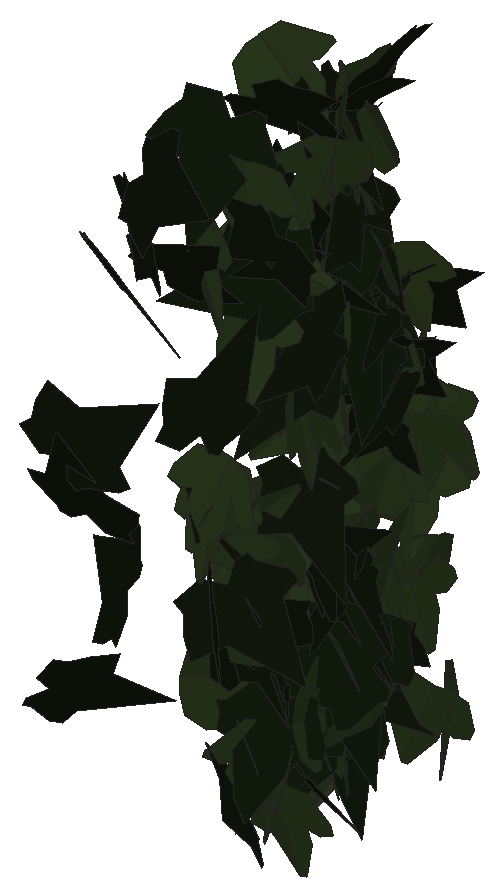
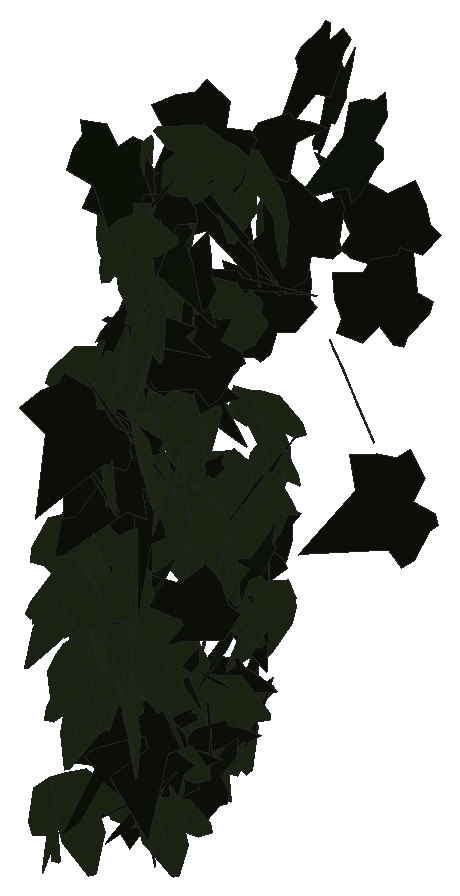
# SketchUp Ruby script. Lengths in inches.
U = 1.inch
M = Sketchup.active_model
def pt(a) = Geom::Point3d.new(a.map { |v| v * U })
def face(e, loops, mat)
  f = e.add_face(loops[0].map { |a| pt(a) })
  loops[1..].each { |l| e.add_face(l.map { |a| pt(a) }).erase! }
  f.material = f.back_material = mat if mat
  f
end
# faces: each face lists its corners as indices into pts; further lists are holes
def faces(e, pts, list, mat = nil) = list.each { |f| face(e, (f[0].is_a?(Array) ? f : [f]).map { |l| l.map { |i| pts[i] } }, mat) }
# xy, xz, yz: faces in a plane at the given z, y or x. An outline is a flat list of corners, or four numbers for a rectangle; further outlines are holes
def ring(l) = l.size == 4 ? [[l[0], l[1]], [l[2], l[1]], [l[2], l[3]], [l[0], l[3]]] : l.each_slice(2).to_a
def flat(e, list, mat, &to3) = list.each { |f| face(e, (f[0].is_a?(Array) ? f : [f]).map { |l| ring(l).map { |u, v| to3.(u, v) } }, mat) }
def xy(e, z, list, mat = nil) = flat(e, list, mat) { |x, y| [x, y, z] }
def xz(e, y, list, mat = nil) = flat(e, list, mat) { |x, z| [x, y, z] }
def yz(e, x, list, mat = nil) = flat(e, list, mat) { |y, z| [x, y, z] }
def lines(e, pts, list) = list.each { |a, b| e.add_line(pt(pts[a]), pt(pts[b])) }
# prism: a flat outline (further loops are holes) pulled along v
def prism(e, loops, v, mat = nil)
  f = face(e, loops, mat); d = Geom::Vector3d.new(v.map { |x| x * U })
  f.pushpull(f.normal.samedirection?(d) ? d.length : -d.length)
end
def box(e, o, s, mat = nil) = prism(e, [[o, [o[0] + s[0], o[1], o[2]], [o[0] + s[0], o[1] + s[1], o[2]], [o[0], o[1] + s[1], o[2]]]], [0, 0, s[2]], mat)
def at(x, y, z, deg = 0) = Geom::Transformation.translation(pt([x, y, z])) * Geom::Transformation.rotation(ORIGIN, Z_AXIS, deg.degrees)
def axes(o, x, y, z) = Geom::Transformation.new([*x, 0, *y, 0, *z, 0, *pt(o).to_a, 1])
def part(name) = M.definitions.add(name)
# library, detail: a bought-in or finely detailed component or shape, given as its bounding box
def library(name, o, s) = part(name).tap { |d| box(d.entities, o, s) }
def detail(e, o, s) = box(e.add_group.entities, o, s)
def put(e, d, t, mat = nil) = e.add_instance(d, t).tap { |i| i.material = mat if mat }
def group(e, t, mat = nil) = e.add_group.tap { |g| g.transformation = t; g.material = mat if mat }.entities
root = M.entities
M.materials.add("efeu1").color = [18, 25, 13]
M.materials.add("efeu2").color = [43, 57, 29]
c1 = part("ivyleaf_9")
p = [[1.54,2.16,1.25],[1.36,2.04,1.19],[-0.21,0.99,0.68],[-0.71,1.11,0.82],[-0.85,0.86,0.67],[-0.8,0.17,0.21],
  [-0.9,-0.01,0.1],[-0.67,-0.16,-0.02],[-0.08,-0.08,-0.05],[-0.03,-0.6,-0.4],[0.65,-0.88,-0.66],[0.83,-0.6,-0.49],
  [1.29,-0.42,-0.43],[1.8125,-0.07,-0.26],[1.21,0.44,0.15]]
faces(c1.entities,p,[[0,1,2,3,4,5,6,7,8,9,10,11,12,13,14]],"efeu1")
c2 = part("ivyleaf_10")
p = [[0,0.5,-0.03],[-0.0625,2.02,-0.43],[-0.19,2.01,-0.46],[-0.54,1.05,-0.29],[-0.52,0.625,-0.18],[-0.83,0.76,-0.28],
  [-1.16,0.64,-0.33],[-1.15,0.33,-0.24],[-0.77,-0.39,0.02],[-0.3,-0.51,0.16],[0.04,-0.48,0.23],[-0.02,2.01,-0.4375],
  [-0.06,2.01,-0.43],[0.04,-0.49,0.23],[0.67,-0.49,0.14],[1.38,0.36,-0.2],[1.375,0.51,-0.24],[0.81,0.65,-0.19],
  [0.62,0.59,-0.15],[0.6,1.09,-0.28],[0.5,1.23,-0.31]]
faces(c2.entities,p,[[0,1,2,3,4,5,6,7,8,9,10],[11,12,0,13,14,15,16,17,18,19,20]],"efeu2")
put(root,c1,axes([54.05,220.4,216.4],[0.34278,0.22043,0.28967],[0.24301,0.15765,-0.40754],[-0.27101,0.42018,0.00094]))
put(root,c2,axes([54.22,224.41,218.67],[-0.03576,-0.11891,-0.48434],[0.01811,-0.48557,0.11788],[-0.49839,-0.00912,0.03904]))
put(root,c2,axes([54.375,225.42,215.87],[0.18568,-0.42925,-0.17682],[-0.07392,0.16068,-0.46767],[0.45832,0.19982,-0.00379]))
put(root,c2,axes([54.09,224.46,218.04],[-0.36251,-0.05995,-0.33911],[0.33393,0.05912,-0.36742],[0.08415,-0.49286,-0.00282]))
put(root,c2,axes([54.24,224.94,214.08],[0.46856,0.17151,-0.03227],[-0.02948,-0.01334,-0.49895],[-0.17201,0.46948,-0.00239]))
put(root,c2,axes([54.38,223.75,215.08],[-0.39712,-0.30366,0.00943],[-0.00588,-0.00784,-0.4999],[0.30375,-0.39715,0.00266]))
put(root,c2,axes([54.36,225.33,217.76],[0.03123,-0.49331,-0.0753],[-0.0092,0.07486,-0.49428],[0.49894,0.03226,-0.0044]))
put(root,c2,axes([54.4,224.6,218.3],[0.11142,0.20479,-0.44232],[-0.22127,-0.38303,-0.23308],[-0.43431,0.24769,0.00527]))
put(root,c2,axes([54.35,225.23,219.43],[0.23453,-0.43827,-0.05396],[-0.02651,0.04701,-0.49708],[0.44079,0.23602,-0.00119]))
put(root,c2,axes([54.34,226.05,217.52],[0.20141,-0.37178,0.26687],[-0.13467,0.23051,0.42276],[-0.43738,-0.24217,-0.00728]))
put(root,c2,axes([54.39,225.23,216.52],[-0.02085,-0.4841,0.12333],[-0.0114,-0.12294,-0.48452],[0.49944,-0.02301,-0.00591]))
put(root,c2,axes([54.14,223.17,217.26],[-0.11766,-0.20198,0.44199],[0.19181,0.39854,0.23319],[-0.4465,0.22443,-0.01631]))
put(root,c2,axes([54.01,223.77,220.5625],[0.23375,0.17848,0.40436],[0.33446,0.22761,-0.29381],[-0.28895,0.40784,-0.01298]))
put(root,c1,axes([54.26,224.69,216.43],[0.31553,-0.2274,-0.31422],[-0.24211,0.20099,-0.38857],[0.30303,0.39736,0.01672]))
put(root,c2,axes([54.36,222.51,215.71],[-0.02289,0.15784,0.47388],[-0.09692,0.46396,-0.15922],[-0.48998,-0.09914,0.00936]))
put(root,c1,axes([54.02,222.37,220.75],[0.47903,0.08705,-0.11382],[0.11154,0.02279,0.48687],[0.08995,-0.49184,0.00241]))
put(root,c2,axes([54.33,225.03,220.95],[-0.43291,0.2453,-0.04912],[0.03857,-0.03155,-0.49751],[-0.24718,-0.43455,0.0084]))
put(root,c2,axes([54.34,225.08,220.54],[-0.35128,0.35581,-0.00154],[0.00098,-0.00119,-0.5],[-0.35581,-0.35128,0.00014]))
put(root,c2,axes([54.25,224.82,216.13],[0.296,0.40228,0.02356],[0.01311,0.0196,-0.49944],[-0.40276,0.29629,0.00105]))
put(root,c2,axes([54.41,225.33,222.08],[-0.08046,-0.49329,-0.01376],[0.0058,0.01299,-0.4998],[0.49345,-0.08059,0.00363]))
put(root,c2,axes([54.27,223.07,217.87],[0.4921,-0.06748,0.0573],[0.05604,-0.01301,-0.49668],[0.06852,0.49525,-0.00524]))
put(root,c1,axes([54.1875,223.01,217.86],[0.25765,-0.39361,-0.16937],[-0.09192,0.14226,-0.47044],[0.41853,0.27356,0.00094]))
put(root,c2,axes([54.36,224.77,215.36],[0.39361,-0.30823,0.00803],[0.00619,-0.00511,-0.49994],[0.30827,0.39366,-0.0002]))
put(root,c1,axes([54.09,223.44,216.71],[0.10994,-0.30855,0.37777],[0.18723,-0.33089,-0.32475],[0.4504,0.21287,0.04278]))
put(root,c2,axes([54.38,224.76,219.52],[0.45695,-0.2011,-0.02755],[-0.02422,0.01338,-0.49923],[0.20153,0.45758,0.00249]))
put(root,c2,axes([54.71,223.45,217.19],[-0.33889,0.00409,0.36761],[-0.36707,0.02391,-0.33866],[-0.02035,-0.49941,-0.0132]))
put(root,c2,axes([54.28,224.91,218.7],[-0.28279,0.31307,-0.26836],[0.16132,-0.21547,-0.42136],[-0.37948,-0.3249,0.02085]))
put(root,c1,axes([54.12,224.02,220.1875],[0.45448,0.092,0.18703],[0.18277,0.03976,-0.46369],[-0.10019,0.48985,0.00251]))
put(root,c2,axes([54.55,223.54,216.52],[0.41301,0.10931,-0.25976],[-0.25932,-0.03304,-0.42622],[-0.11035,0.48678,0.02941]))
put(root,c1,axes([54.55,225.14,215.3],[0.24453,0.30102,-0.31558],[-0.19954,-0.24449,-0.38782],[-0.3878,0.31561,0.00056]))
put(root,c1,axes([54.14,221.01,221.62],[0.44584,-0.22613,0.00938],[0.009,-0.00299,-0.49991],[0.22615,0.44593,0.00141]))
put(root,c2,axes([54.34,224.8,214.75],[0.46124,0.19179,0.02185],[0.0202,0.00831,-0.49952],[-0.19197,0.46168,-0.00008]))
put(root,c1,axes([54.4,224.21,214.64],[-0.23472,-0.43944,-0.04236],[0.01747,0.03869,-0.49819],[0.44113,-0.23536,-0.00281]))
put(root,c1,axes([54.4,222.96,222.46],[-0.24192,-0.43704,-0.0218],[0.01226,0.01813,-0.49952],[0.43741,-0.24222,0.00194]))
put(root,c2,axes([54.1875,224,222.79],[0.29809,0.25187,0.31257],[0.23027,0.21161,-0.39012],[-0.32881,0.37654,0.01016]))
put(root,c2,axes([54.73,223.16,214.08],[-0.10513,0.1466,-0.46632],[-0.30733,0.3511,0.17966],[0.38013,0.3244,0.01629]))
put(root,c2,axes([54.6,223.45,216.71],[-0.25815,0.31504,0.29001],[-0.21702,0.19567,-0.40573],[-0.36914,-0.33535,0.03571]))
put(root,c1,axes([54.08,224.46,216.34],[0.0728,-0.12051,0.47977],[0.47761,-0.10914,-0.09988],[0.1288,0.47283,0.09922]))
put(root,c2,axes([54.15,223.83,220.46],[-0.18991,-0.09297,-0.45309],[0.45939,0.01905,-0.19646],[0.05379,-0.49091,0.07818]))
put(root,c2,axes([54.23,224.48,217.92],[-0.03627,0.08339,-0.49166],[0.26295,-0.41566,-0.08989],[-0.42373,-0.26508,-0.01371]))
put(root,c2,axes([54.5625,225.32,216.375],[-0.40626,0.26631,0.11845],[-0.10087,0.06217,-0.48576],[-0.27345,-0.41859,0.00322]))
put(root,c1,axes([54.125,223.99,214.19],[0.40948,-0.22122,0.18272],[0.16269,-0.08325,-0.4654],[0.23634,0.4406,0.00381]))
put(root,c2,axes([54.22,225.14,214.05],[0.12176,-0.17351,0.45284],[0.38666,-0.24706,-0.19863],[0.29269,0.39856,0.07402]))
put(root,c2,axes([54.47,224.65,214.2],[0.4326,-0.2507,0.00346],[0.00858,0.00791,-0.49986],[0.25057,0.43254,0.01115]))
put(root,c1,axes([54.3125,225.13,214.84],[0.03126,-0.19052,-0.46122],[0.05316,0.46077,-0.18673],[0.49618,-0.03736,0.04907]))
put(root,c1,axes([54.33,224.99,214.23],[0.10204,-0.48631,-0.05561],[-0.0161,0.05344,-0.49687],[0.48921,0.10319,-0.00475]))
put(root,c1,axes([54.47,220.4,218.77],[0.44084,-0.13651,0.19241],[-0.17838,0.07399,0.4612],[-0.15439,-0.47528,0.01653]))
put(root,c2,axes([54.57,224.58,221.12],[0.03468,-0.44069,0.23365],[0.0145,-0.23322,-0.44204],[0.49859,0.03743,-0.0034]))
put(root,c1,axes([54.31,223.49,215.83],[0.31074,-0.38547,-0.06968],[-0.0482,0.05064,-0.49509],[0.38874,0.3144,-0.00569]))
put(root,c2,axes([54.59,223.3,214.69],[-0.09554,-0.46012,0.17075],[0.0057,-0.17499,-0.46834],[0.49075,-0.08755,0.03868]))
put(root,c1,axes([54.8,224.47,221.74],[-0.28188,0.38157,-0.15795],[0.00994,-0.18491,-0.46444],[-0.41285,-0.26498,0.09666]))
put(root,c1,axes([54.79,224.75,220.54],[-0.47448,-0.12463,0.09664],[-0.08407,-0.05934,-0.4893],[0.13343,-0.48057,0.03536]))
put(root,c1,axes([54.61,224.75,214.58],[-0.35998,-0.34674,-0.01344],[0.00803,0.01105,-0.49981],[0.34691,-0.36007,-0.00239]))
put(root,c1,axes([54.26,224.29,220.82],[0.03748,-0.09754,0.48896],[0.24863,-0.42137,-0.10312],[0.43218,0.25087,0.01692]))
put(root,c2,axes([54.33,226.07,217.6875],[0.39812,0.15768,0.25815],[0.22894,0.12182,-0.42749],[-0.19771,0.45858,0.0248]))
put(root,c2,axes([54.57,224.3,214.5],[-0.30713,0.39347,0.0293],[-0.0099,0.02944,-0.49903],[-0.39443,-0.30711,-0.0103]))
put(root,c1,axes([54.74,225.03,218.1],[0.29054,0.13382,-0.38429],[-0.35796,-0.14052,-0.31956],[-0.19353,0.46081,0.01415]))
put(root,c1,axes([54.93,223.37,220.52],[-0.43058,0.03863,0.25121],[-0.24767,-0.17477,-0.39763],[0.05709,-0.46686,0.16964]))
put(root,c2,axes([54.5,222.55,218.06],[0.45547,-0.18474,0.09177],[0.08639,-0.03114,-0.49149],[0.18731,0.46357,0.00355]))
put(root,c2,axes([54.73,223.82,217.58],[-0.35171,-0.30861,0.17624],[-0.07583,-0.17707,-0.46141],[0.3472,-0.35129,0.07775]))
put(root,c1,axes([54.95,220.5,217.91],[-0.24316,0.06039,-0.4327],[-0.42377,0.08783,0.2504],[0.10625,0.48851,0.00847]))
put(root,c2,axes([54.47,222.44,221.24],[-0.34459,0.19538,-0.3051],[0.19029,-0.2607,-0.38187],[-0.3083,-0.37929,0.1053]))
put(root,c1,axes([54.47,223.76,214.41],[-0.09208,0.17408,0.45958],[0.07637,-0.45683,0.18834],[0.48548,0.10488,0.05754]))
put(root,c1,axes([54.82,223.23,221.52],[-0.48442,0.08746,-0.08767],[0.08628,-0.01555,-0.49225],[-0.08883,-0.49205,-0.00003]))
put(root,c2,axes([54.59,223.18,219.98],[0.11338,0.47158,-0.12149],[-0.01833,-0.12052,-0.48491],[-0.48663,0.11441,-0.01004]))
put(root,c2,axes([54.73,222.91,221.92],[-0.49218,-0.08157,0.03326],[-0.02091,-0.07519,-0.49387],[0.08557,-0.48754,0.0706]))
put(root,c2,axes([54.57,223.95,217.48],[0.33575,0.37041,0.0084],[0.00544,0.00641,-0.49993],[-0.37046,0.3358,0.00028]))
put(root,c2,axes([54.71,222.43,218.39],[0.48226,-0.05939,-0.1179],[-0.11397,0.03811,-0.48534],[0.06663,0.495,0.02323]))
put(root,c1,axes([54.83,222.93,216.45],[0.05816,0.37791,-0.32219],[-0.03354,-0.32066,-0.38217],[-0.49547,0.06607,-0.01195]))
put(root,c1,axes([54.97,224.91,219.11],[-0.49277,0.01681,0.08302],[-0.08318,-0.00351,-0.49302],[-0.016,-0.4997,0.00625]))
put(root,c1,axes([54.87,224.42,222.27],[0.08065,0.49279,-0.02561],[-0.08062,-0.01244,-0.4933],[-0.48682,0.08369,0.07745]))
put(root,c2,axes([54.55,222.74,217.36],[-0.07303,-0.34382,0.35561],[0.15711,0.32472,0.34622],[-0.46902,0.16231,0.0606]))
put(root,c2,axes([54.87,223.78,218.82],[-0.44899,0.15129,0.15976],[-0.16193,0.01861,-0.47269],[-0.14897,-0.4762,0.03228]))
put(root,c1,axes([54.87,225.09,218.75],[0.00131,0.40428,-0.2942],[0.00271,-0.2942,-0.40428],[-0.49999,-0.00054,-0.00296]))
put(root,c1,axes([55,224.23,216.24],[-0.3561,0.35087,0.00887],[-0.00433,0.00823,-0.49991],[-0.35096,-0.35612,-0.00282]))
put(root,c2,axes([54.67,222.8,216.375],[0.10149,0.08171,-0.48273],[0.13234,0.47006,0.10739],[0.47137,-0.14957,0.07378]))
put(root,c2,axes([54.79,224.54,221.91],[-0.37735,0.32437,0.04889],[-0.06386,0.00045,-0.4959],[-0.32176,-0.3805,0.04109]))
put(root,c1,axes([54.88,223.82,219.37],[-0.47802,-0.13718,-0.05174],[0.04832,0.0192,-0.49729],[0.13842,-0.48043,-0.0051]))
put(root,c1,axes([54.52,221.3,221.93],[0.0508,-0.2309,0.44057],[0.08486,-0.43235,-0.23637],[0.49012,0.09879,-0.00474]))
put(root,c1,axes([54.53,224.78,214.97],[0.05599,-0.48439,-0.11059],[0.06436,0.11742,-0.48174],[0.49267,0.03971,0.0755]))
put(root,c1,axes([54.57,223.35,222.66],[0.44446,0.21621,0.07555],[0.06051,0.04822,-0.49398],[-0.22089,0.44825,0.0167]))
put(root,c1,axes([54.77,221.08,222.75],[0.12822,-0.08386,-0.47595],[-0.30237,0.37021,-0.14668],[0.37701,0.32544,0.04423]))
put(root,c1,axes([54.6,224.36,222.29],[0.27378,-0.36773,-0.19954],[-0.10014,0.17394,-0.45795],[0.40622,0.29072,0.02159]))
put(root,c1,axes([54.98,221.98,217.11],[0.13555,-0.03482,-0.48001],[-0.46921,0.10138,-0.13986],[0.10707,0.48837,-0.00519]))
put(root,c2,axes([55.07,224.82,221.61],[-0.32038,0.16716,-0.34556],[-0.30332,0.16562,0.36134],[0.23527,0.44117,-0.00472]))
put(root,c2,axes([54.625,224.51,221.21],[0.29075,-0.27638,0.29846],[0.23188,-0.1888,-0.40073],[0.3342,0.37144,0.01838]))
put(root,c1,axes([55.08,224.98,219.54],[-0.4158,0.27608,0.02984],[-0.02824,0.01141,-0.49907],[-0.27625,-0.41671,0.0061]))
put(root,c1,axes([54.83,223.34,215.15],[-0.39352,-0.27415,-0.14137],[0.12097,0.07363,-0.47953],[0.28374,-0.41161,0.00838]))
put(root,c2,axes([54.74,226.16,217.46],[-0.07757,-0.42921,-0.24446],[0.17826,0.20645,-0.41905],[0.46066,-0.15216,0.12099]))
put(root,c2,axes([54.84,225.25,217.31],[-0.05237,-0.45798,-0.19368],[0.06803,0.18632,-0.45897],[0.49258,-0.07442,0.04279]))
put(root,c1,axes([54.67,222.87,214.03],[-0.0954,-0.14452,0.46906],[0.1002,-0.47351,-0.12551],[0.48048,0.07005,0.11931]))
put(root,c1,axes([54.53,220.03,219.66],[-0.07323,0.00384,0.49459],[0.45799,-0.18827,0.06927],[0.18677,0.46318,0.02406]))
put(root,c2,axes([54.86,223.67,218.8],[-0.11957,0.48415,0.03613],[-0.05589,0.02324,-0.49632],[-0.48226,-0.12273,0.04856]))
put(root,c2,axes([54.86,225.32,218.86],[-0.42479,0.24224,-0.10429],[0.02427,-0.16097,-0.47276],[-0.26262,-0.4067,0.125]))
put(root,c1,axes([54.74,224.72,220.83],[0.17807,-0.3675,-0.28851],[-0.13714,0.25404,-0.40824],[0.44664,0.22452,-0.01033]))
put(root,c2,axes([54.88,224.94,220.26],[-0.37657,0.32886,0.00669],[-0.00749,0.0016,-0.49994],[-0.32884,-0.37663,0.00372]))
put(root,c1,axes([54.81,225.01,218.73],[0.305,0.385,0.09353],[0.05752,0.07376,-0.49117],[-0.392,0.31038,0.0007]))
put(root,c2,axes([55.08,225.66,214.32],[-0.42451,-0.17102,0.20135],[-0.18091,-0.08952,-0.45745],[0.19251,-0.46124,0.01413]))
put(root,c1,axes([54.65,224.375,216.3],[0.37783,-0.32142,-0.06272],[-0.04545,0.04337,-0.49604],[0.32431,0.38054,0.00356]))
put(root,c2,axes([54.84,225.24,217.37],[-0.30142,-0.35568,-0.18066],[0.16551,0.09453,-0.46225],[0.36298,-0.33846,0.06076]))
put(root,c2,axes([54.88,224.23,215.54],[-0.3746,0.32882,-0.03938],[0.03741,-0.01707,-0.49831],[-0.32905,-0.37628,-0.01182]))
put(root,c1,axes([54.75,222.57,216.93],[-0.02643,-0.24534,-0.43487],[0.04258,0.43278,-0.24675],[0.49748,-0.05008,-0.00198]))
put(root,c1,axes([54.84,221.98,219.23],[-0.11085,-0.18715,0.45021],[0.35136,0.28943,0.20683],[-0.33802,0.36223,0.06735]))
put(root,c1,axes([54.96,224.77,215.58],[-0.32202,-0.38211,0.01702],[-0.00438,-0.01857,-0.49964],[0.38247,-0.32194,0.00861]))
put(root,c2,axes([54.92,225.51,215.77],[-0.17986,-0.4483,-0.12915],[0.1104,0.09358,-0.4786],[0.45328,-0.20068,0.06532]))
put(root,c2,axes([55.02,225.64,216.14],[-0.04931,-0.46861,0.16726],[-0.00976,-0.16714,-0.47114],[0.49747,-0.04972,0.00734]))
put(root,c2,axes([55.09,223.95,221.88],[-0.25409,-0.39927,0.1613],[-0.08678,-0.13597,-0.47327],[0.42179,-0.2685,-0.0002]))
put(root,c1,axes([54.92,225.36,219.5],[0.28481,0.40466,0.07162],[0.03623,0.06208,-0.49481],[-0.40935,0.28704,0.00604]))
put(root,c2,axes([54.99,223.18,214.11],[-0.4988,0.02413,-0.02476],[0.02488,0.00198,-0.49938],[-0.024,-0.49941,-0.00317]))
put(root,c1,axes([55.14,224.64,222.73],[-0.04151,0.49531,0.05425],[-0.01307,0.05334,-0.49698],[-0.4981,-0.04268,0.00852]))
put(root,c2,axes([54.96,225.24,216.61],[0.20546,-0.44081,0.11607],[0.0552,-0.10232,-0.4863],[0.45248,0.21265,0.00662]))
put(root,c2,axes([54.97,225.18,219.99],[-0.45371,-0.17541,-0.11568],[0.10829,0.04068,-0.48643],[0.18006,-0.46645,0.00108]))
put(root,c1,axes([55.27,222.69,221.46],[0.11829,0.14865,-0.46251],[-0.42432,-0.20018,-0.17286],[-0.23656,0.43339,0.07879]))
put(root,c2,axes([55.07,225.44,217.81],[-0.44581,-0.22612,0.01108],[-0.01266,0.00046,-0.49984],[0.22604,-0.44595,-0.00614]))
put(root,c1,axes([54.88,224.99,219.3125],[-0.05386,-0.49539,0.04103],[-0.01205,-0.03996,-0.49825],[0.49695,-0.05466,-0.00763]))
put(root,c2,axes([54.875,224.37,222.36],[0.30168,-0.31568,0.2436],[0.18059,-0.16417,-0.43639],[0.3555,0.35128,0.01496]))
put(root,c1,axes([54.84,223.74,217.86],[0.09738,-0.44911,-0.19703],[-0.03206,0.19462,-0.45945],[0.48938,0.10211,0.00911]))
put(root,c1,axes([55.16,225.11,218.63],[-0.43591,0.16588,-0.18017],[0.15292,-0.10295,-0.46478],[-0.19129,-0.46031,0.03902]))
put(root,c2,axes([55.06,224.55,214.79],[-0.05719,-0.47014,-0.16031],[0.01305,0.15989,-0.47357],[0.49655,-0.05835,-0.00602]))
put(root,c2,axes([55,225.52,217.1875],[0.12901,0.47751,-0.07308],[-0.06869,-0.05674,-0.492],[-0.47816,0.13699,0.05095]))
put(root,c1,axes([54.74,224.58,216.65],[0.26527,-0.41701,0.07575],[0.04493,-0.06119,-0.4942],[0.42144,0.269,0.005]))
put(root,c2,axes([55,226.08,214.28],[-0.24569,0.38165,-0.20971],[0.00222,-0.23969,-0.4388],[-0.43547,-0.21655,0.11608]))
put(root,c1,axes([55.29,223.64,219.84],[-0.46931,0.17205,-0.01215],[0.00909,-0.01051,-0.49981],[-0.17224,-0.46935,0.00674]))
put(root,c2,axes([55.2,223.31,215.09],[-0.09273,0.12634,0.47481],[-0.26656,0.39296,-0.15662],[-0.41273,-0.28218,-0.00552]))
put(root,c2,axes([55.02,223.16,214.62],[0.34892,-0.3573,0.02437],[0.02328,-0.01133,-0.49933],[0.35737,0.34959,0.00873]))
put(root,c1,axes([55.43,224.11,215.52],[-0.4023,0.03569,0.29475],[-0.2956,-0.00161,-0.40326],[-0.02784,-0.49872,0.02239]))
